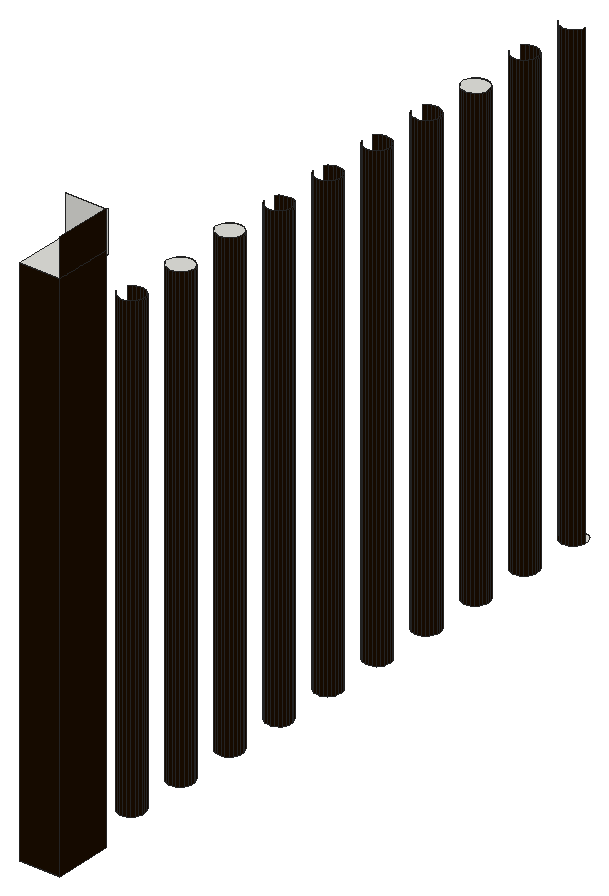
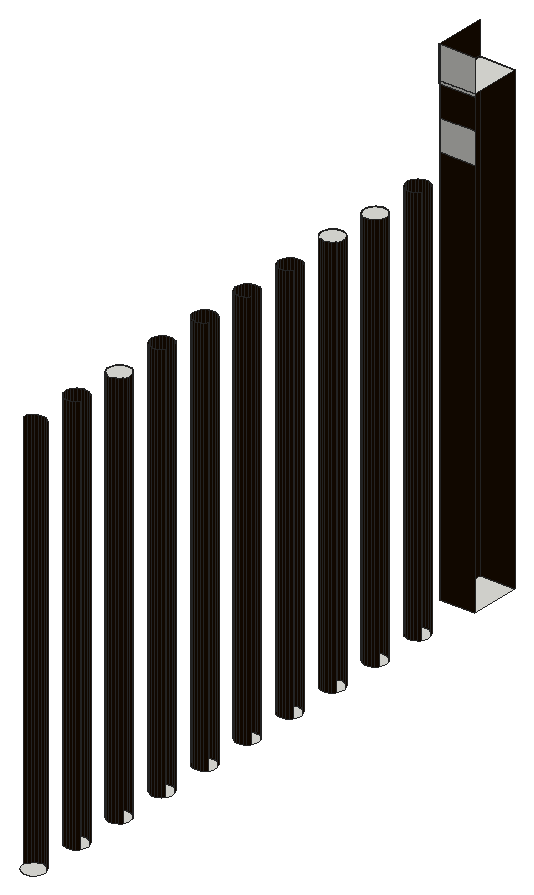
# SketchUp Ruby script. Lengths in inches.
U = 1.inch
M = Sketchup.active_model
def pt(a) = Geom::Point3d.new(a.map { |v| v * U })
def face(e, loops, mat)
  f = e.add_face(loops[0].map { |a| pt(a) })
  loops[1..].each { |l| e.add_face(l.map { |a| pt(a) }).erase! }
  f.material = f.back_material = mat if mat
  f
end
# faces: each face lists its corners as indices into pts; further lists are holes
def faces(e, pts, list, mat = nil) = list.each { |f| face(e, (f[0].is_a?(Array) ? f : [f]).map { |l| l.map { |i| pts[i] } }, mat) }
# xy, xz, yz: faces in a plane at the given z, y or x. An outline is a flat list of corners, or four numbers for a rectangle; further outlines are holes
def ring(l) = l.size == 4 ? [[l[0], l[1]], [l[2], l[1]], [l[2], l[3]], [l[0], l[3]]] : l.each_slice(2).to_a
def flat(e, list, mat, &to3) = list.each { |f| face(e, (f[0].is_a?(Array) ? f : [f]).map { |l| ring(l).map { |u, v| to3.(u, v) } }, mat) }
def xy(e, z, list, mat = nil) = flat(e, list, mat) { |x, y| [x, y, z] }
def xz(e, y, list, mat = nil) = flat(e, list, mat) { |x, z| [x, y, z] }
def yz(e, x, list, mat = nil) = flat(e, list, mat) { |y, z| [x, y, z] }
def lines(e, pts, list) = list.each { |a, b| e.add_line(pt(pts[a]), pt(pts[b])) }
# prism: a flat outline (further loops are holes) pulled along v
def prism(e, loops, v, mat = nil)
  f = face(e, loops, mat); d = Geom::Vector3d.new(v.map { |x| x * U })
  f.pushpull(f.normal.samedirection?(d) ? d.length : -d.length)
end
def box(e, o, s, mat = nil) = prism(e, [[o, [o[0] + s[0], o[1], o[2]], [o[0] + s[0], o[1] + s[1], o[2]], [o[0], o[1] + s[1], o[2]]]], [0, 0, s[2]], mat)
def at(x, y, z, deg = 0) = Geom::Transformation.translation(pt([x, y, z])) * Geom::Transformation.rotation(ORIGIN, Z_AXIS, deg.degrees)
def axes(o, x, y, z) = Geom::Transformation.new([*x, 0, *y, 0, *z, 0, *pt(o).to_a, 1])
def part(name) = M.definitions.add(name)
# library, detail: a bought-in or finely detailed component or shape, given as its bounding box
def library(name, o, s) = part(name).tap { |d| box(d.entities, o, s) }
def detail(e, o, s) = box(e.add_group.entities, o, s)
def put(e, d, t, mat = nil) = e.add_instance(d, t).tap { |i| i.material = mat if mat }
def group(e, t, mat = nil) = e.add_group.tap { |g| g.transformation = t; g.material = mat if mat }.entities
root = M.entities
M.materials.add("[Metal Seamed]1").color = [28, 14, 0]
xy(root,618.25,[[361.97,67.28,366.15,73.28],[363.55,78.41,363.21,78.5,362.92,78.67,362.67,78.91,362.5,79.21,362.41,79.54,362.41,79.88,362.5,80.21,362.67,80.51,362.91,80.75,363.2,80.92,363.54,81.01,363.88,81.01,364.21,80.93,364.51,80.76,364.75,80.51,364.92,80.22,365.01,79.89,365.01,79.55,364.93,79.21,364.76,78.92,364.51,78.67,364.22,78.5,363.89,78.41],[363.55,84.85,363.21,84.94,362.92,85.11,362.67,85.35,362.5,85.64,362.41,85.97,362.41,86.32,362.5,86.65,362.67,86.94,362.91,87.1875,363.2,87.36,363.54,87.45,363.88,87.45,364.21,87.36,364.51,87.19,364.75,86.95,364.92,86.66,365.01,86.33,365.01,85.98,364.93,85.65,364.76,85.35,364.51,85.11,364.22,84.9375,363.89,84.85],[363.55,91.29,363.21,91.37,362.92,91.54,362.67,91.78,362.5,92.08,362.41,92.41,362.41,92.75,362.5,93.08,362.67,93.38,362.91,93.625,363.2,93.8,363.54,93.89,363.88,93.89,364.21,93.8,364.51,93.63,364.75,93.39,364.92,93.09,365.01,92.76,365.01,92.42,364.93,92.09,364.76,91.79,364.51,91.55,364.22,91.375,363.89,91.29],[363.55,97.72,363.21,97.81,362.92,97.98,362.67,98.22,362.5,98.52,362.41,98.85,362.41,99.19,362.5,99.52,362.67,99.82,362.91,100.0625,363.2,100.24,363.54,100.33,363.88,100.33,364.21,100.24,364.51,100.07,364.75,99.83,364.92,99.53,365.01,99.2,365.01,98.86,364.93,98.53,364.76,98.23,364.51,97.99,364.22,97.8125,363.89,97.72],
  [363.55,104.16,363.21,104.25,362.92,104.42,362.67,104.66,362.5,104.96,362.41,105.29,362.41,105.63,362.5,105.96,362.67,106.26,362.91,106.5,363.2,106.67,363.54,106.76,363.88,106.76,364.21,106.68,364.51,106.51,364.75,106.26,364.92,105.97,365.01,105.64,365.01,105.3,364.93,104.96,364.76,104.67,364.51,104.42,364.22,104.25,363.89,104.16],[363.55,110.6,363.21,110.69,362.92,110.86,362.67,111.1,362.5,111.39,362.41,111.72,362.41,112.07,362.5,112.4,362.67,112.69,362.91,112.9375,363.2,113.11,363.54,113.2,363.88,113.2,364.21,113.11,364.51,112.94,364.75,112.7,364.92,112.41,365.01,112.08,365.01,111.73,364.93,111.4,364.76,111.1,364.51,110.86,364.22,110.6875,363.89,110.6],[363.55,117.04,363.21,117.12,362.92,117.29,362.67,117.53,362.5,117.83,362.41,118.16,362.41,118.5,362.5,118.83,362.67,119.13,362.91,119.375,363.2,119.55,363.54,119.64,363.88,119.64,364.21,119.55,364.51,119.38,364.75,119.14,364.92,118.84,365.01,118.51,365.01,118.17,364.93,117.84,364.76,117.54,364.51,117.3,364.22,117.125,363.89,117.04],[363.55,123.47,363.21,123.56,362.92,123.73,362.67,123.97,362.5,124.27,362.41,124.6,362.41,124.94,362.5,125.27,362.67,125.57,362.91,125.8125,363.2,125.99,363.54,126.08,363.88,126.08,364.21,125.99,364.51,125.82,364.75,125.58,364.92,125.28,365.01,124.95,365.01,124.61,364.93,124.28,364.76,123.98,364.51,123.74,364.22,123.5625,363.89,123.47],[363.55,129.91,363.21,130,362.92,130.17,362.67,130.41,362.5,130.71,362.41,131.04,362.41,131.38,362.5,131.71,362.67,132.01,362.91,132.25,363.2,132.42,363.54,132.51,363.88,132.51,364.21,132.43,364.51,132.26,364.75,132.01,364.92,131.72,365.01,131.39,365.01,131.05,364.93,130.71,364.76,130.42,364.51,130.17,364.22,130,363.89,129.91],
  [363.55,136.35,363.21,136.44,362.92,136.61,362.67,136.85,362.5,137.14,362.41,137.47,362.41,137.82,362.5,138.15,362.67,138.44,362.91,138.6875,363.2,138.86,363.54,138.95,363.88,138.95,364.21,138.86,364.51,138.69,364.75,138.45,364.92,138.16,365.01,137.83,365.01,137.48,364.93,137.15,364.76,136.85,364.51,136.61,364.22,136.4375,363.89,136.35]])
xy(root,666.375,[[363.55,123.47,363.89,123.47,364.22,123.5625,364.51,123.74,364.76,123.98,364.93,124.28,365.01,124.61,365.01,124.95,364.92,125.28,364.75,125.58,364.51,125.82,364.21,125.99,363.88,126.08,363.54,126.08,363.2,125.99,362.91,125.8125,362.67,125.57,362.5,125.27,362.41,124.94,362.41,124.6,362.5,124.27,362.67,123.97,362.92,123.73,363.21,123.56]])
xy(root,666.5625,[[363.55,84.85,363.89,84.85,364.22,84.9375,364.51,85.11,364.76,85.35,364.93,85.65,365.01,85.98,365.01,86.33,364.92,86.66,364.75,86.95,364.51,87.19,364.21,87.36,363.88,87.45,363.54,87.45,363.2,87.36,362.91,87.1875,362.67,86.94,362.5,86.65,362.41,86.32,362.41,85.97,362.5,85.64,362.67,85.35,362.92,85.11,363.21,84.94]])
xy(root,666.9375,[[363.55,91.29,363.89,91.29,364.22,91.375,364.51,91.55,364.76,91.79,364.93,92.09,365.01,92.42,365.01,92.76,364.92,93.09,364.75,93.39,364.51,93.63,364.21,93.8,363.88,93.89,363.54,93.89,363.2,93.8,362.91,93.625,362.67,93.38,362.5,93.08,362.41,92.75,362.41,92.41,362.5,92.08,362.67,91.78,362.92,91.54,363.21,91.37]])
xy(root,674.375,[[361.97,67.28,366.15,73.28]])
xz(root,67.28,[[361.97,618.25,366.15,674.375]],"[Metal Seamed]1")
xz(root,73.28,[[361.98,666.66,366.15,670.37],[361.97,674.05,366.15,674.375],[366.15,674.05,366.34,678.3125],[361.97,674.375,366.15,678.3125]])
xz(root,73.28,[[361.97,618.25,366.15,666.66],[361.97,670.37,366.15,674.05]],"[Metal Seamed]1")
xz(root,78.41,[[363.55,618.25,363.89,666.66]],"[Metal Seamed]1")
xz(root,81.01,[[363.54,618.25,363.88,666.66]],"[Metal Seamed]1")
xz(root,84.85,[[363.55,618.25,363.89,666.5625]],"[Metal Seamed]1")
xz(root,87.45,[[363.54,618.25,363.88,666.5625]],"[Metal Seamed]1")
xz(root,91.29,[[363.55,618.25,363.89,666.9375]],"[Metal Seamed]1")
xz(root,93.89,[[363.54,618.25,363.88,666.9375]],"[Metal Seamed]1")
xz(root,97.72,[[363.55,618.25,363.89,666.66]],"[Metal Seamed]1")
xz(root,100.33,[[363.54,618.25,363.88,666.66]],"[Metal Seamed]1")
xz(root,104.16,[[363.55,618.25,363.89,666.66]],"[Metal Seamed]1")
xz(root,106.76,[[363.54,618.25,363.88,666.66]],"[Metal Seamed]1")
xz(root,110.6,[[363.55,618.25,363.89,666.66]],"[Metal Seamed]1")
xz(root,113.2,[[363.54,618.25,363.88,666.66]],"[Metal Seamed]1")
xz(root,117.04,[[363.55,618.25,363.89,666.66]],"[Metal Seamed]1")
xz(root,119.64,[[363.54,618.25,363.88,666.66]],"[Metal Seamed]1")
xz(root,123.47,[[363.55,618.25,363.89,666.375]],"[Metal Seamed]1")
xz(root,126.08,[[363.54,618.25,363.88,666.375]],"[Metal Seamed]1")
xz(root,129.91,[[363.55,618.25,363.89,666.66]],"[Metal Seamed]1")
xz(root,132.51,[[363.54,618.25,363.88,666.66]],"[Metal Seamed]1")
xz(root,136.35,[[363.55,618.25,363.89,666.66]],"[Metal Seamed]1")
yz(root,365.01,[[79.55,618.25,79.89,666.66],[85.98,618.25,86.33,666.5625],[92.42,618.25,92.76,666.9375],[98.86,618.25,99.2,666.66],[105.3,618.25,105.64,666.66],
  [111.73,618.25,112.08,666.66],[118.17,618.25,118.51,666.66],[124.61,618.25,124.95,666.375],[131.05,618.25,131.39,666.66]],"[Metal Seamed]1")
yz(root,366.15,[[67.28,618.25,73.28,674.375],[67.28,674.375,73.28,678.3125]],"[Metal Seamed]1")
p = [[363.21,78.5,618.25],[363.55,78.41,618.25],[363.55,78.41,666.66],[363.21,78.5,666.66],[363.89,78.41,618.25],[364.22,78.5,618.25],
  [364.22,78.5,666.66],[363.89,78.41,666.66],[362.92,78.67,618.25],[362.92,78.67,666.66],[364.51,78.67,618.25],[364.51,78.67,666.66],
  [362.67,78.91,618.25],[362.67,78.91,666.66],[364.76,78.92,618.25],[364.76,78.92,666.66],[362.5,79.21,618.25],[362.5,79.21,666.66],
  [364.93,79.21,618.25],[364.93,79.21,666.66],[365.01,79.55,618.25],[365.01,79.55,666.66],[365.01,79.89,618.25],[364.92,80.22,618.25],
  [364.92,80.22,666.66],[365.01,79.89,666.66],[364.75,80.51,618.25],[364.75,80.51,666.66],[362.91,80.75,618.25],[362.67,80.51,618.25],
  [362.67,80.51,666.66],[362.91,80.75,666.66],[364.51,80.76,618.25],[364.51,80.76,666.66],[363.2,80.92,618.25],[363.2,80.92,666.66],
  [364.21,80.93,618.25],[364.21,80.93,666.66],[363.54,81.01,618.25],[363.54,81.01,666.66],[363.88,81.01,618.25],[363.88,81.01,666.66],
  [363.21,84.94,618.25],[363.55,84.85,618.25],[363.55,84.85,666.5625],[363.21,84.94,666.5625],[363.89,84.85,618.25],[364.22,84.9375,618.25],
  [364.22,84.9375,666.5625],[363.89,84.85,666.5625],[362.92,85.11,618.25],[362.92,85.11,666.5625],[364.51,85.11,618.25],[364.51,85.11,666.5625],
  [362.67,85.35,618.25],[362.67,85.35,666.5625],[364.76,85.35,618.25],[364.76,85.35,666.5625],[362.5,85.64,618.25],[362.5,85.64,666.5625],
  [364.93,85.65,618.25],[364.93,85.65,666.5625],[365.01,85.98,618.25],[365.01,85.98,666.5625],[365.01,86.33,618.25],[364.92,86.66,618.25],
  [364.92,86.66,666.5625],[365.01,86.33,666.5625],[364.75,86.95,618.25],[364.75,86.95,666.5625],[362.91,87.1875,618.25],[362.67,86.94,618.25],
  [362.67,86.94,666.5625],[362.91,87.1875,666.5625],[364.51,87.19,618.25],[364.51,87.19,666.5625],[363.2,87.36,618.25],[363.2,87.36,666.5625],
  [364.21,87.36,618.25],[364.21,87.36,666.5625],[363.54,87.45,618.25],[363.54,87.45,666.5625],[363.88,87.45,618.25],[363.88,87.45,666.5625],
  [363.21,91.37,618.25],[363.55,91.29,618.25],[363.55,91.29,666.9375],[363.21,91.37,666.9375],[363.89,91.29,618.25],[364.22,91.375,618.25],
  [364.22,91.375,666.9375],[363.89,91.29,666.9375],[362.92,91.54,618.25],[362.92,91.54,666.9375],[364.51,91.55,618.25],[364.51,91.55,666.9375],
  [362.67,91.78,618.25],[362.67,91.78,666.9375],[364.76,91.79,618.25],[364.76,91.79,666.9375],[362.5,92.08,618.25],[362.5,92.08,666.9375],
  [364.93,92.09,618.25],[364.93,92.09,666.9375],[365.01,92.42,618.25],[365.01,92.42,666.9375],[365.01,92.76,618.25],[364.92,93.09,618.25],
  [364.92,93.09,666.9375],[365.01,92.76,666.9375],[364.75,93.39,618.25],[364.75,93.39,666.9375],[362.91,93.625,618.25],[362.67,93.38,618.25],
  [362.67,93.38,666.9375],[362.91,93.625,666.9375],[364.51,93.63,618.25],[364.51,93.63,666.9375],[363.2,93.8,618.25],[363.2,93.8,666.9375],
  [364.21,93.8,618.25],[364.21,93.8,666.9375],[363.54,93.89,618.25],[363.54,93.89,666.9375],[363.88,93.89,618.25],[363.88,93.89,666.9375],
  [363.21,97.81,618.25],[363.55,97.72,618.25],[363.55,97.72,666.66],[363.21,97.81,666.66],[363.89,97.72,618.25],[364.22,97.8125,618.25],
  [364.22,97.8125,666.66],[363.89,97.72,666.66],[362.92,97.98,618.25],[362.92,97.98,666.66],[364.51,97.99,618.25],[364.51,97.99,666.66],
  [362.67,98.22,618.25],[362.67,98.22,666.66],[364.76,98.23,618.25],[364.76,98.23,666.66],[362.5,98.52,618.25],[362.5,98.52,666.66],
  [364.93,98.53,618.25],[364.93,98.53,666.66],[365.01,98.86,618.25],[365.01,98.86,666.66],[365.01,99.2,618.25],[364.92,99.53,618.25],
  [364.92,99.53,666.66],[365.01,99.2,666.66],[364.75,99.83,618.25],[364.75,99.83,666.66],[362.91,100.0625,618.25],[362.67,99.82,618.25],
  [362.67,99.82,666.66],[362.91,100.0625,666.66],[364.51,100.07,618.25],[364.51,100.07,666.66],[363.2,100.24,618.25],[363.2,100.24,666.66],
  [364.21,100.24,618.25],[364.21,100.24,666.66],[363.54,100.33,618.25],[363.54,100.33,666.66],[363.88,100.33,618.25],[363.88,100.33,666.66],
  [362.92,104.42,618.25],[363.21,104.25,618.25],[363.21,104.25,666.66],[362.92,104.42,666.66],[363.55,104.16,618.25],[363.55,104.16,666.66],
  [363.89,104.16,618.25],[364.22,104.25,618.25],[364.22,104.25,666.66],[363.89,104.16,666.66],[364.51,104.42,618.25],[364.51,104.42,666.66],
  [362.67,104.66,618.25],[362.67,104.66,666.66],[364.76,104.67,618.25],[364.76,104.67,666.66],[362.5,104.96,618.25],[362.5,104.96,666.66],
  [364.93,104.96,618.25],[364.93,104.96,666.66],[365.01,105.3,618.25],[365.01,105.3,666.66],[365.01,105.64,618.25],[364.92,105.97,618.25],
  [364.92,105.97,666.66],[365.01,105.64,666.66],[364.75,106.26,618.25],[364.75,106.26,666.66],[362.91,106.5,618.25],[362.67,106.26,618.25],
  [362.67,106.26,666.66],[362.91,106.5,666.66],[364.51,106.51,618.25],[364.51,106.51,666.66],[363.2,106.67,618.25],[363.2,106.67,666.66],
  [364.21,106.68,618.25],[364.21,106.68,666.66],[363.54,106.76,618.25],[363.54,106.76,666.66],[363.88,106.76,618.25],[363.88,106.76,666.66],
  [363.21,110.69,618.25],[363.55,110.6,618.25],[363.55,110.6,666.66],[363.21,110.69,666.66],[363.89,110.6,618.25],[364.22,110.6875,618.25],
  [364.22,110.6875,666.66],[363.89,110.6,666.66],[362.92,110.86,618.25],[362.92,110.86,666.66],[364.51,110.86,618.25],[364.51,110.86,666.66],
  [362.67,111.1,618.25],[362.67,111.1,666.66],[364.76,111.1,618.25],[364.76,111.1,666.66],[362.5,111.39,618.25],[362.5,111.39,666.66],
  [364.93,111.4,618.25],[364.93,111.4,666.66],[365.01,111.73,618.25],[365.01,111.73,666.66],[365.01,112.08,618.25],[364.92,112.41,618.25],
  [364.92,112.41,666.66],[365.01,112.08,666.66],[364.75,112.7,618.25],[364.75,112.7,666.66],[362.91,112.9375,618.25],[362.67,112.69,618.25],
  [362.67,112.69,666.66],[362.91,112.9375,666.66],[364.51,112.94,618.25],[364.51,112.94,666.66],[363.2,113.11,618.25],[363.2,113.11,666.66],
  [364.21,113.11,618.25],[364.21,113.11,666.66],[363.54,113.2,618.25],[363.54,113.2,666.66],[363.88,113.2,618.25],[363.88,113.2,666.66],
  [363.21,117.12,618.25],[363.55,117.04,618.25],[363.55,117.04,666.66],[363.21,117.12,666.66],[363.89,117.04,618.25],[364.22,117.125,618.25],
  [364.22,117.125,666.66],[363.89,117.04,666.66],[362.92,117.29,618.25],[362.92,117.29,666.66],[364.51,117.3,618.25],[364.51,117.3,666.66],
  [362.67,117.53,618.25],[362.67,117.53,666.66],[364.76,117.54,618.25],[364.76,117.54,666.66],[362.5,117.83,618.25],[362.5,117.83,666.66],
  [364.93,117.84,618.25],[364.93,117.84,666.66],[365.01,118.17,618.25],[365.01,118.17,666.66],[365.01,118.51,618.25],[364.92,118.84,618.25],
  [364.92,118.84,666.66],[365.01,118.51,666.66],[364.75,119.14,618.25],[364.75,119.14,666.66],[362.91,119.375,618.25],[362.67,119.13,618.25],
  [362.67,119.13,666.66],[362.91,119.375,666.66],[364.51,119.38,618.25],[364.51,119.38,666.66],[363.2,119.55,618.25],[363.2,119.55,666.66],
  [364.21,119.55,618.25],[364.21,119.55,666.66],[363.54,119.64,618.25],[363.54,119.64,666.66],[363.88,119.64,618.25],[363.88,119.64,666.66],
  [363.21,123.56,618.25],[363.55,123.47,618.25],[363.55,123.47,666.375],[363.21,123.56,666.375],[363.89,123.47,618.25],[364.22,123.5625,618.25],
  [364.22,123.5625,666.375],[363.89,123.47,666.375],[362.92,123.73,618.25],[362.92,123.73,666.375],[364.51,123.74,618.25],[364.51,123.74,666.375],
  [362.67,123.97,618.25],[362.67,123.97,666.375],[364.76,123.98,618.25],[364.76,123.98,666.375],[362.5,124.27,618.25],[362.5,124.27,666.375],
  [364.93,124.28,618.25],[364.93,124.28,666.375],[365.01,124.61,618.25],[365.01,124.61,666.375],[365.01,124.95,618.25],[364.92,125.28,618.25],
  [364.92,125.28,666.375],[365.01,124.95,666.375],[364.75,125.58,618.25],[364.75,125.58,666.375],[362.91,125.8125,618.25],[362.67,125.57,618.25],
  [362.67,125.57,666.375],[362.91,125.8125,666.375],[364.51,125.82,618.25],[364.51,125.82,666.375],[363.2,125.99,618.25],[363.2,125.99,666.375],
  [364.21,125.99,618.25],[364.21,125.99,666.375],[363.54,126.08,618.25],[363.54,126.08,666.375],[363.88,126.08,618.25],[363.88,126.08,666.375],
  [363.21,130,618.25],[363.55,129.91,618.25],[363.55,129.91,666.66],[363.21,130,666.66],[363.89,129.91,618.25],[364.22,130,618.25],
  [364.22,130,666.66],[363.89,129.91,666.66],[362.92,130.17,618.25],[362.92,130.17,666.66],[364.51,130.17,618.25],[364.51,130.17,666.66],
  [362.67,130.41,618.25],[362.67,130.41,666.66],[364.76,130.42,618.25],[364.76,130.42,666.66],[362.5,130.71,618.25],[362.5,130.71,666.66],
  [364.93,130.71,618.25],[364.93,130.71,666.66],[365.01,131.05,618.25],[365.01,131.05,666.66],[365.01,131.39,618.25],[364.92,131.72,618.25],
  [364.92,131.72,666.66],[365.01,131.39,666.66],[364.75,132.01,618.25],[364.75,132.01,666.66],[362.91,132.25,618.25],[362.67,132.01,618.25],
  [362.67,132.01,666.66],[362.91,132.25,666.66],[364.51,132.26,618.25],[364.51,132.26,666.66],[363.2,132.42,618.25],[363.2,132.42,666.66],
  [364.21,132.43,618.25],[364.21,132.43,666.66],[363.54,132.51,618.25],[363.54,132.51,666.66],[363.88,132.51,618.25],[363.88,132.51,666.66],
  [363.21,136.44,618.25],[363.55,136.35,618.25],[363.55,136.35,666.66],[363.21,136.44,666.66],[363.89,136.35,618.25],[364.22,136.4375,618.25],
  [364.22,136.4375,666.66],[363.89,136.35,666.66],[362.92,136.61,618.25],[362.92,136.61,666.66],[364.51,136.61,618.25],[364.51,136.61,666.66],
  [362.67,136.85,618.25],[362.67,136.85,666.66],[364.76,136.85,618.25],[364.76,136.85,666.66],[362.5,137.14,618.25],[362.5,137.14,666.66],
  [364.93,137.15,618.25],[364.93,137.15,666.66],[365.01,137.48,618.25],[365.01,137.48,666.66]]
faces(root,p,[[0,1,2,3],[4,5,6,7],[8,0,3,9],[5,10,11,6],[12,8,9,13],[10,14,15,11],[16,12,13,17],[14,18,19,15],
  [18,20,21,19],[22,23,24,25],[23,26,27,24],[28,29,30,31],[26,32,33,27],[34,28,31,35],[32,36,37,33],[38,34,35,39],
  [36,40,41,37],[42,43,44,45],[46,47,48,49],[50,42,45,51],[47,52,53,48],[54,50,51,55],[52,56,57,53],[58,54,55,59],
  [56,60,61,57],[60,62,63,61],[64,65,66,67],[65,68,69,66],[70,71,72,73],[68,74,75,69],[76,70,73,77],[74,78,79,75],
  [80,76,77,81],[78,82,83,79],[84,85,86,87],[88,89,90,91],[92,84,87,93],[89,94,95,90],[96,92,93,97],[94,98,99,95],
  [100,96,97,101],[98,102,103,99],[102,104,105,103],[106,107,108,109],[107,110,111,108],[112,113,114,115],[110,116,117,111],[118,112,115,119],
  [116,120,121,117],[122,118,119,123],[120,124,125,121],[126,127,128,129],[130,131,132,133],[134,126,129,135],[131,136,137,132],[138,134,135,139],
  [136,140,141,137],[142,138,139,143],[140,144,145,141],[144,146,147,145],[148,149,150,151],[149,152,153,150],[154,155,156,157],[152,158,159,153],
  [160,154,157,161],[158,162,163,159],[164,160,161,165],[162,166,167,163],[168,169,170,171],[169,172,173,170],[174,175,176,177],[175,178,179,176],
  [180,168,171,181],[178,182,183,179],[184,180,181,185],[182,186,187,183],[186,188,189,187],[190,191,192,193],[191,194,195,192],[196,197,198,199],
  [194,200,201,195],[202,196,199,203],[200,204,205,201],[206,202,203,207],[204,208,209,205],[210,211,212,213],[214,215,216,217],[218,210,213,219],
  [215,220,221,216],[222,218,219,223],[220,224,225,221],[226,222,223,227],[224,228,229,225],[228,230,231,229],[232,233,234,235],[233,236,237,234],
  [238,239,240,241],[236,242,243,237],[244,238,241,245],[242,246,247,243],[248,244,245,249],[246,250,251,247],[252,253,254,255],[256,257,258,259],
  [260,252,255,261],[257,262,263,258],[264,260,261,265],[262,266,267,263],[268,264,265,269],[266,270,271,267],[270,272,273,271],[274,275,276,277],
  [275,278,279,276],[280,281,282,283],[278,284,285,279],[286,280,283,287],[284,288,289,285],[290,286,287,291],[288,292,293,289],[294,295,296,297],
  [298,299,300,301],[302,294,297,303],[299,304,305,300],[306,302,303,307],[304,308,309,305],[310,306,307,311],[308,312,313,309],[312,314,315,313],
  [316,317,318,319],[317,320,321,318],[322,323,324,325],[320,326,327,321],[328,322,325,329],[326,330,331,327],[332,328,329,333],[330,334,335,331],
  [336,337,338,339],[340,341,342,343],[344,336,339,345],[341,346,347,342],[348,344,345,349],[346,350,351,347],[352,348,349,353],[350,354,355,351],
  [354,356,357,355],[358,359,360,361],[359,362,363,360],[364,365,366,367],[362,368,369,363],[370,364,367,371],[368,372,373,369],[374,370,371,375],
  [372,376,377,373],[378,379,380,381],[382,383,384,385],[386,378,381,387],[383,388,389,384],[390,386,387,391],[388,392,393,389],[394,390,391,395],
  [392,396,397,393],[396,398,399,397]],"[Metal Seamed]1")
